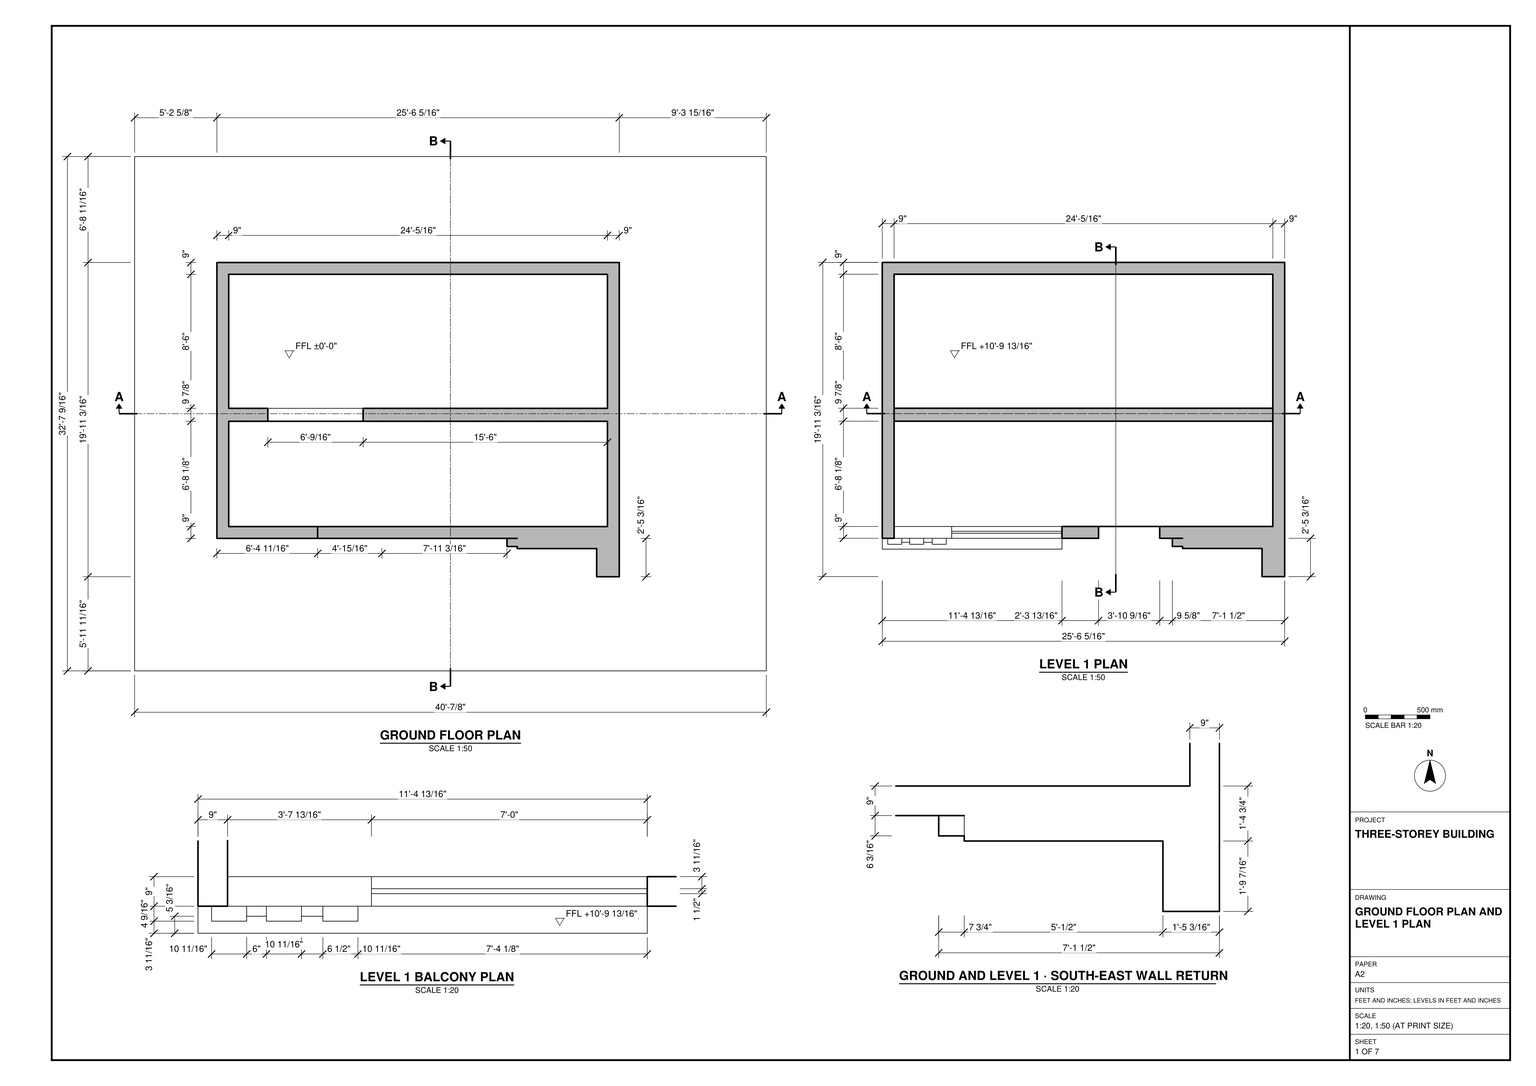
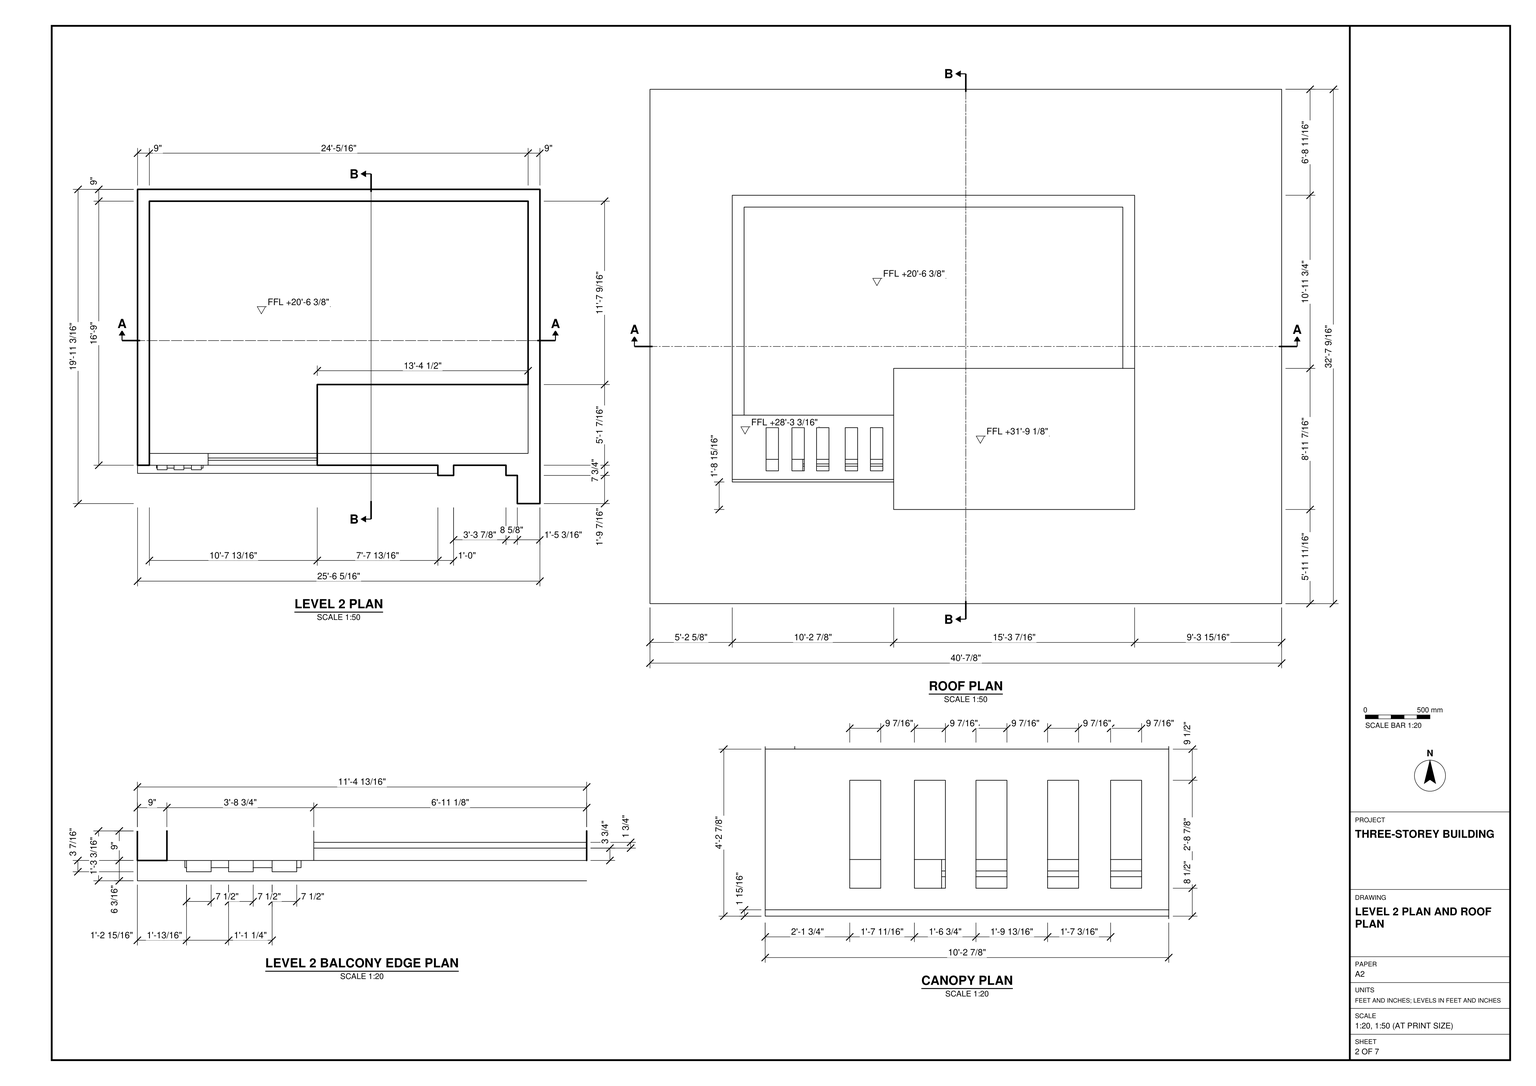
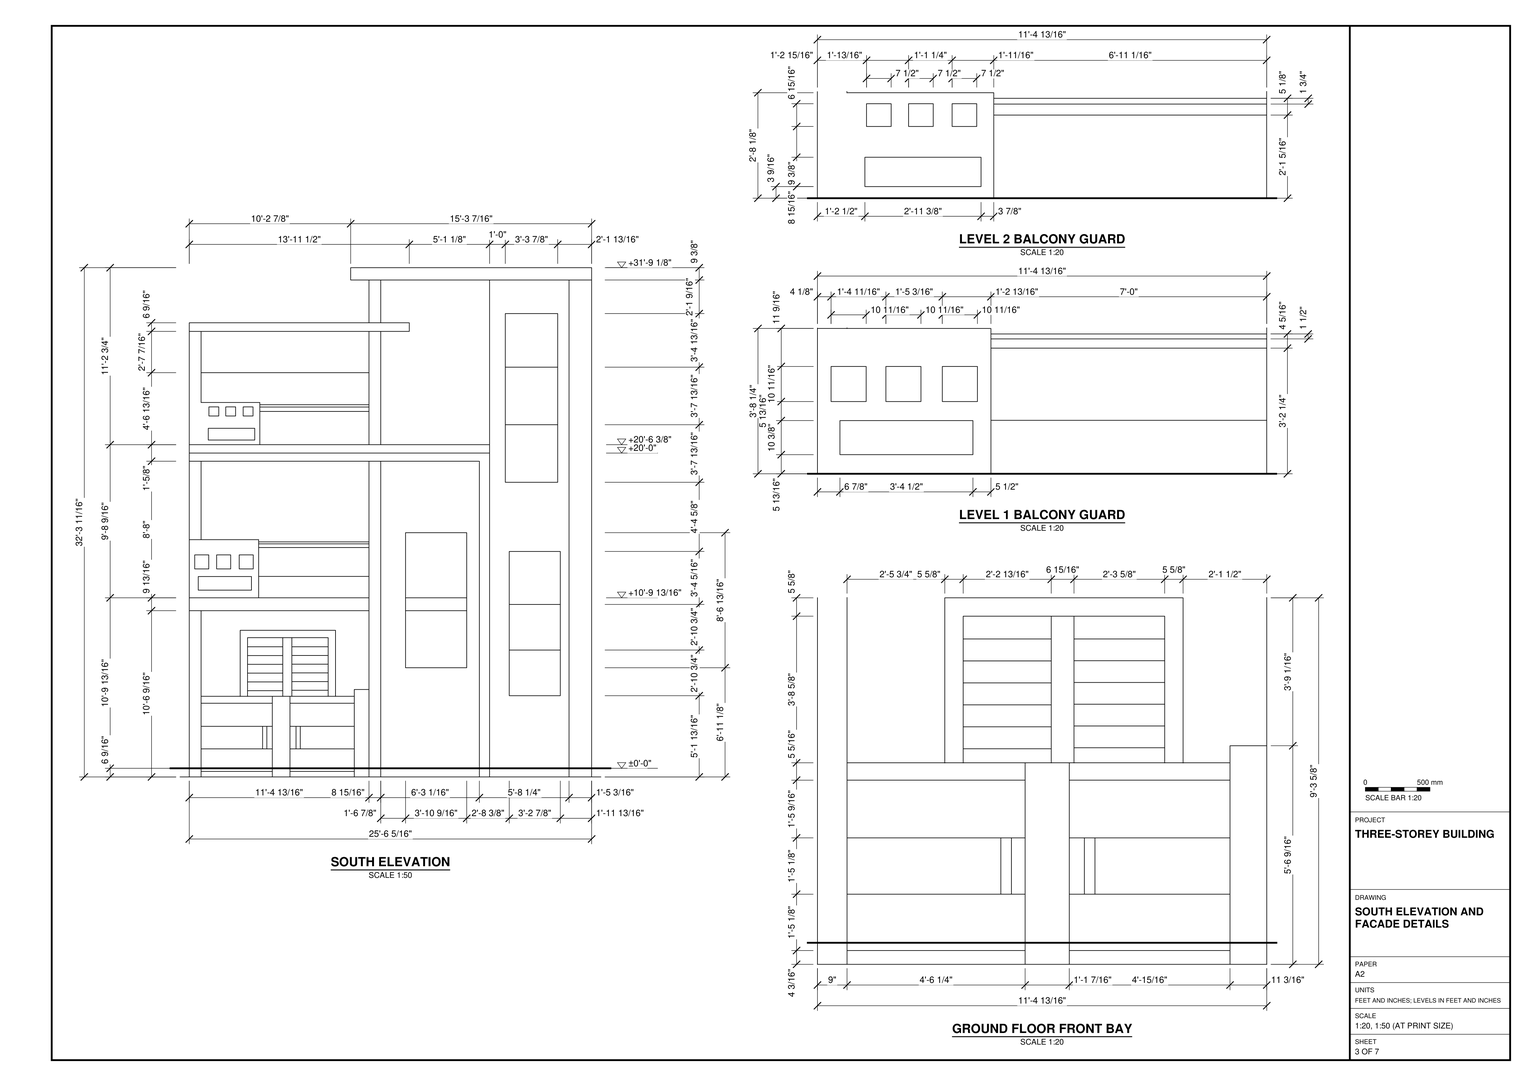
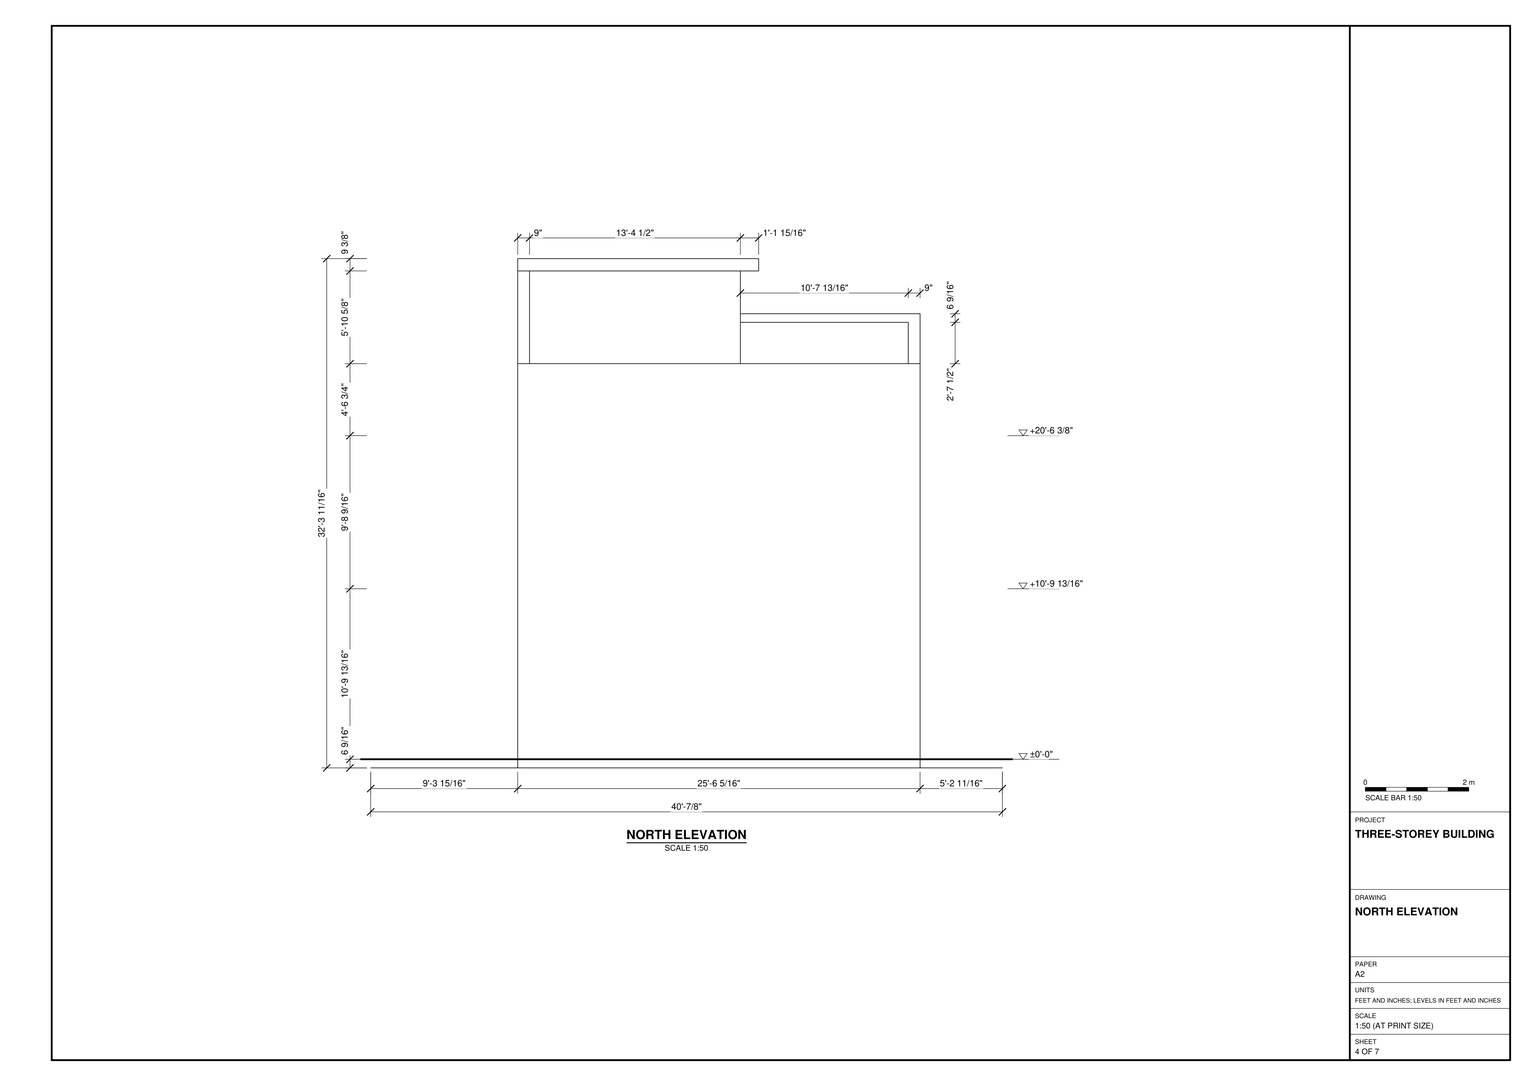
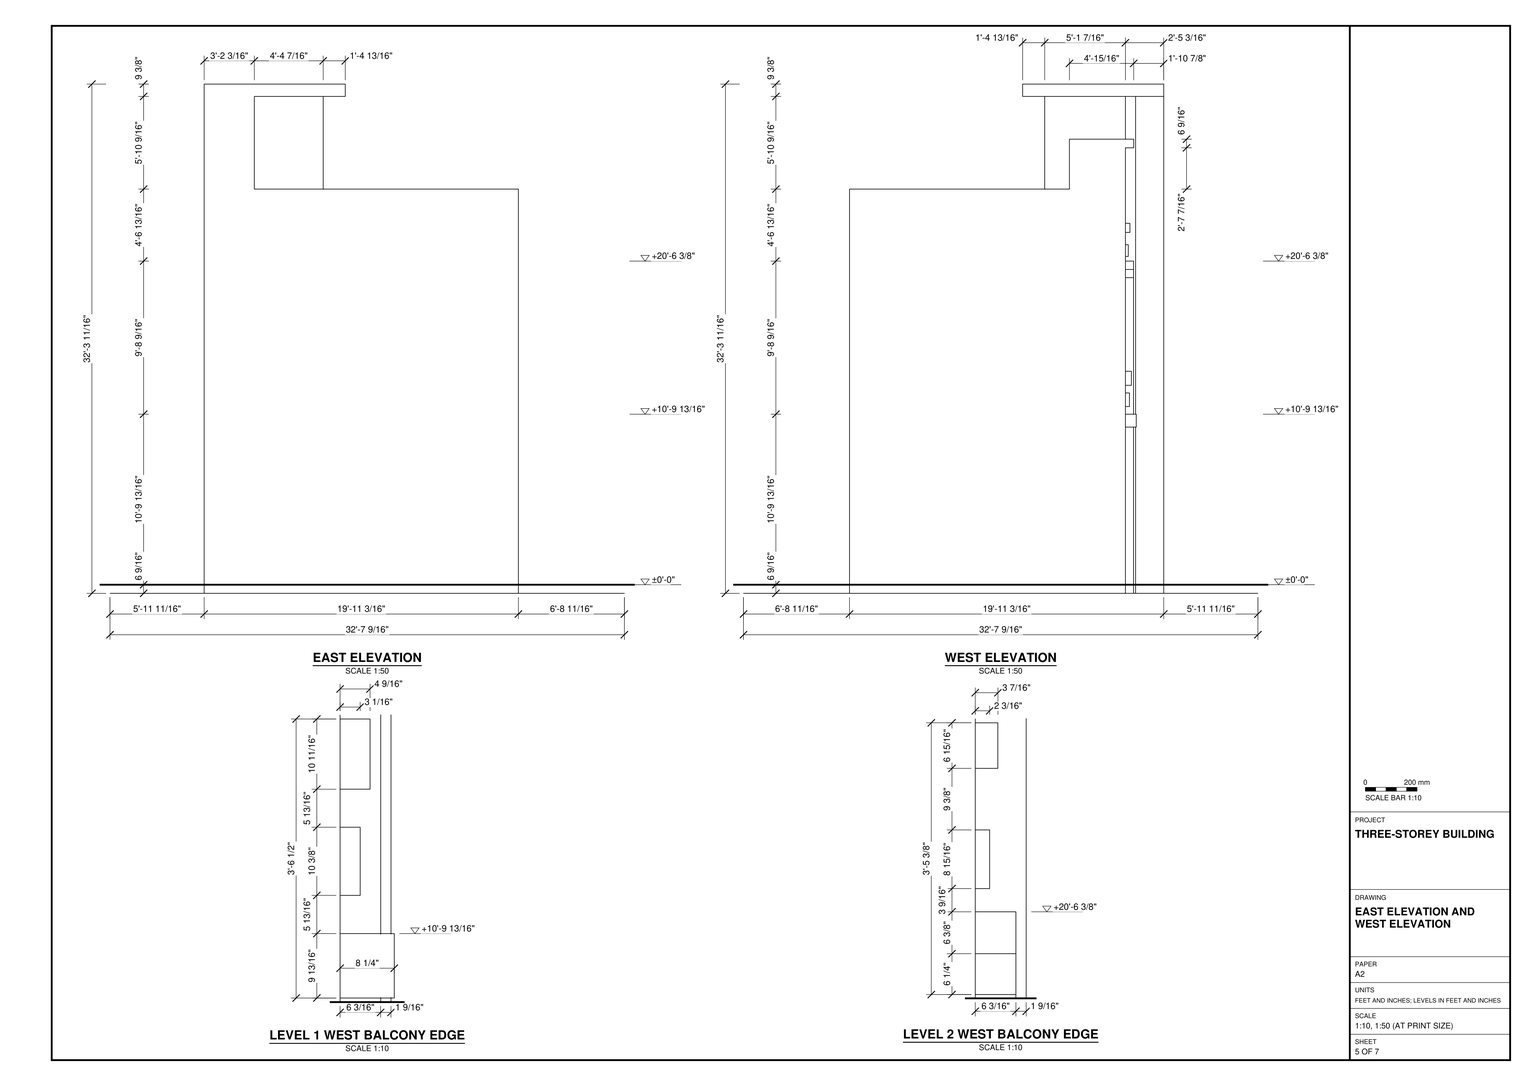
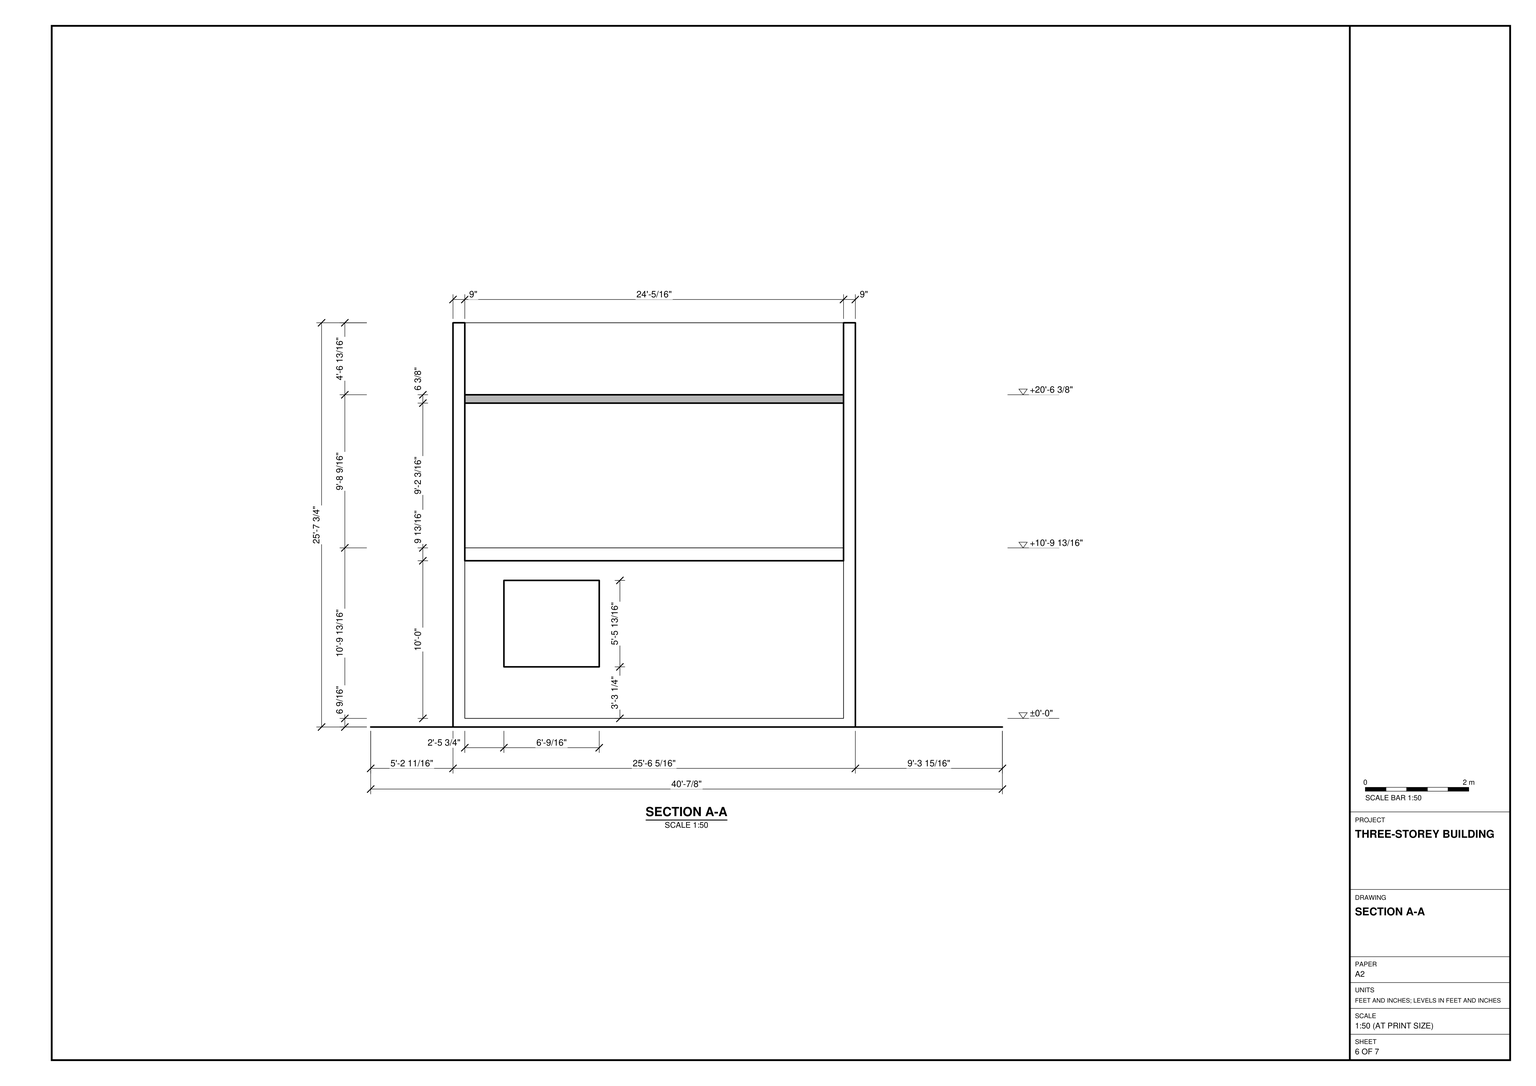
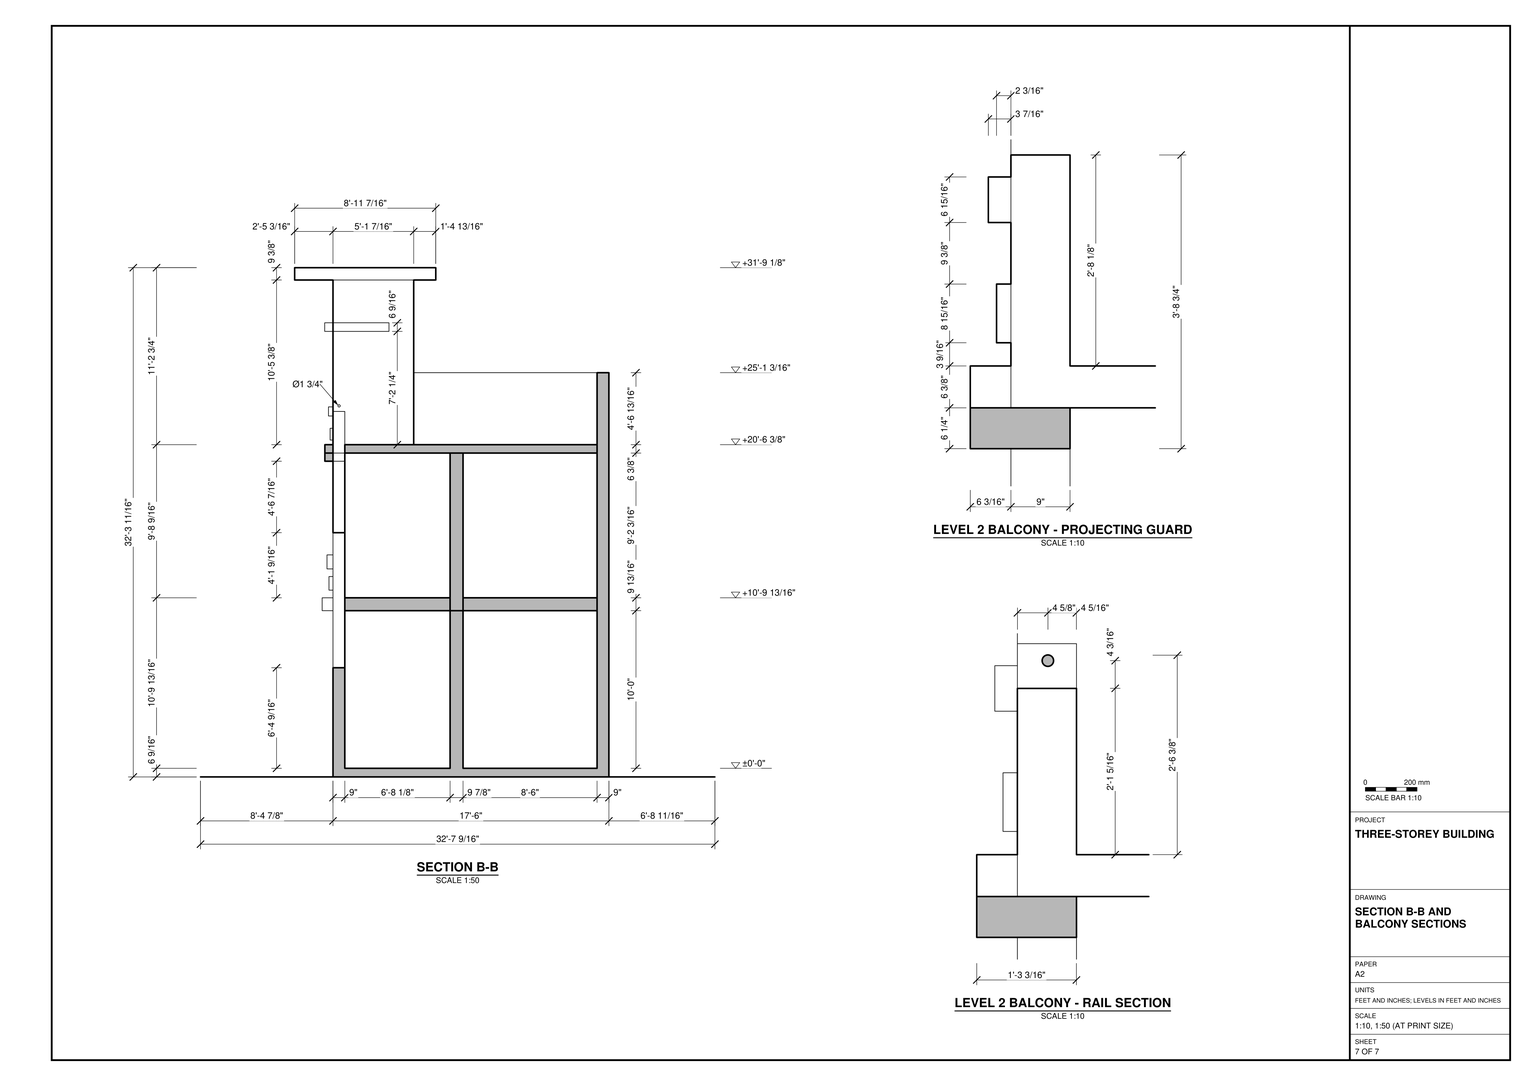
Build the three-storey building in SketchUp from task_files/diagram_01.pdf. Work in feet and inches. The overall model, including the rectangular base, measures 40'-7/8" along X, 32'-7 9/16" along Y and 32'-3 11/16" in height. Set the finished floor levels at ±0'-0", +10'-9 13/16" and +20'-6 3/8".

Position the smaller building footprint on the base using the setbacks on the ground floor plan. Model the floor slabs, perimeter walls and transverse walls at their drawn thicknesses. Keep the passage through the ground floor transverse wall and follow the stepped outline of the south-east wall return. Use the plans and elevations together to locate the openings and distinguish them from surface panels. Include stairs, built-in joinery and main furniture only where shown.

On the south face, align the stacked balconies above the ground floor front bay. Follow the separate guard details for each balcony rather than making the two guards identical. Model the lower slotted canopy and the higher flat roof over the south-east portion, leaving the top floor open where indicated in the roof plan.

Keep walls, slabs and roof elements in separate groups or components, and do the same for each furniture or joinery piece. Use components for repeated parts. Decor and loose items may be any suitable library components. Save one SketchUp model as output_files/three_storey_building_with_balconies_and_slotted_canopy.skp.

# SketchUp Ruby script. Lengths in inches.
U = 1.inch
M = Sketchup.active_model
def pt(a) = Geom::Point3d.new(a.map { |v| v * U })
def face(e, loops, mat)
  f = e.add_face(loops[0].map { |a| pt(a) })
  loops[1..].each { |l| e.add_face(l.map { |a| pt(a) }).erase! }
  f.material = f.back_material = mat if mat
  f
end
# faces: each face lists its corners as indices into pts; further lists are holes
def faces(e, pts, list, mat = nil) = list.each { |f| face(e, (f[0].is_a?(Array) ? f : [f]).map { |l| l.map { |i| pts[i] } }, mat) }
# xy, xz, yz: faces in a plane at the given z, y or x. An outline is a flat list of corners, or four numbers for a rectangle; further outlines are holes
def ring(l) = l.size == 4 ? [[l[0], l[1]], [l[2], l[1]], [l[2], l[3]], [l[0], l[3]]] : l.each_slice(2).to_a
def flat(e, list, mat, &to3) = list.each { |f| face(e, (f[0].is_a?(Array) ? f : [f]).map { |l| ring(l).map { |u, v| to3.(u, v) } }, mat) }
def xy(e, z, list, mat = nil) = flat(e, list, mat) { |x, y| [x, y, z] }
def xz(e, y, list, mat = nil) = flat(e, list, mat) { |x, z| [x, y, z] }
def yz(e, x, list, mat = nil) = flat(e, list, mat) { |y, z| [x, y, z] }
def lines(e, pts, list) = list.each { |a, b| e.add_line(pt(pts[a]), pt(pts[b])) }
# prism: a flat outline (further loops are holes) pulled along v
def prism(e, loops, v, mat = nil)
  f = face(e, loops, mat); d = Geom::Vector3d.new(v.map { |x| x * U })
  f.pushpull(f.normal.samedirection?(d) ? d.length : -d.length)
end
def box(e, o, s, mat = nil) = prism(e, [[o, [o[0] + s[0], o[1], o[2]], [o[0] + s[0], o[1] + s[1], o[2]], [o[0], o[1] + s[1], o[2]]]], [0, 0, s[2]], mat)
def at(x, y, z, deg = 0) = Geom::Transformation.translation(pt([x, y, z])) * Geom::Transformation.rotation(ORIGIN, Z_AXIS, deg.degrees)
def axes(o, x, y, z) = Geom::Transformation.new([*x, 0, *y, 0, *z, 0, *pt(o).to_a, 1])
def part(name) = M.definitions.add(name)
# library, detail: a bought-in or finely detailed component or shape, given as its bounding box
def library(name, o, s) = part(name).tap { |d| box(d.entities, o, s) }
def detail(e, o, s) = box(e.add_group.entities, o, s)
def put(e, d, t, mat = nil) = e.add_instance(d, t).tap { |i| i.material = mat if mat }
def group(e, t, mat = nil) = e.add_group.tap { |g| g.transformation = t; g.material = mat if mat }.entities
root = M.entities
M.materials.add("[Blinds Wood Light]").color = [155, 100, 14]
M.materials.add("[Carpet Diamond Olive]").color = [87, 77, 61]
M.materials.add("[Carpet Plush Charcoal]").color = [87, 87, 87]
M.materials.add("[Color M01]").color = [226, 226, 226]
M.materials.add("[Formica Beige]").color = [132, 117, 93]
M.materials.add("[Formica Beige]1").color = [255, 225, 180]
M.materials.add("[Formica Beige]2").color = [239, 212, 169]
M.materials.add("[Formica Beige]3").color = [211, 187, 149]
M.materials.add("[Formica Graystone]").color = [149, 146, 135]
M.materials.add("[Formica Laminate Dark]").color = [50, 53, 60]
M.materials.add("[Formica Speckled Grey]").color = [94, 105, 111]
M.materials.add("[Stone Masonry Multi]").color = [182, 175, 164]
M.materials.add("[Terrazzo Light Blue]").color = [196, 214, 227]
M.materials.add("[Translucent Glass Blue]").color = [100, 149, 237]
M.materials["[Translucent Glass Blue]"].alpha = 0.5
M.materials.add("[Translucent Glass Safety]").color = [204, 235, 244]
M.materials["[Translucent Glass Safety]"].alpha = 0.5
M.materials.add("[Translucent Glass Sky Reflection]").color = [126, 138, 183]
M.materials["[Translucent Glass Sky Reflection]"].alpha = 0.52
M.materials.add("[Wood Floor Light]").color = [204, 176, 127]
M.materials.add("[Wood Floor Parquet]").color = [145, 89, 39]
M.materials.add("[Wood Veneer 01]").color = [120, 70, 37]
xy(root,0,[[[0,0,480.875,391.5625],[351.76,71.67,368.96,71.67,368.96,310.89,62.65,310.89,62.65,100.86,283.48,100.86,283.48,94.67,291.26,94.67,291.26,93.11,351.76,93.11]],[351.76,71.67,351.76,93.11,291.26,93.11,291.26,100.86,62.65,100.86,62.65,310.89,368.96,310.89,368.96,71.67],[283.48,94.67,291.26,100.86]])
xy(root,6.5625,[[71.65,199.86,359.96,301.89]])
xy(root,6.5625,[[71.65,109.86,359.96,190]],"[Carpet Plush Charcoal]")
xy(root,45.8,[[101.42,190,173.98,199.86]])
xy(root,61.375,[[71.65,100.86,125.88,109.86],[125.88,100.86,139.33,109.86],[139.33,100.86,188.27,109.86]],"[Formica Laminate Dark]")
xy(root,61.83,[[306.24,93.11,345.12,100.86]],"[Formica Speckled Grey]")
xy(root,66.5625,[[188.27,100.86,199.46,109.86]],"[Formica Beige]1")
xy(root,83.12,[[227.29,100.86,273.85,109.86]],"[Formica Beige]")
xy(root,111.62,[[101.42,190,173.98,199.86]])
xy(root,126.5625,[[62.65,92.61,62.65,100.86,71.65,100.86,71.65,109.86,199.46,109.86,199.46,92.61],[71.65,109.86,359.96,190],[71.65,190,359.96,199.86],[71.65,199.86,359.96,301.89]])
xy(root,136.375,[[71.65,199.86,359.96,301.89]])
xy(root,136.375,[[71.65,109.86,359.96,190]],"[Carpet Diamond Olive]")
xy(root,136.375,[[62.65,92.61,199.46,100.86]],"[Formica Beige]1")
xy(root,142.19,[[69.5,97.79,110,100.86]])
xy(root,152.57,[[69.5,97.79,110,100.86]],"[Color M01]")
xy(root,158.36,[[66.8,96.29,77.49,100.86],[83.49,96.29,94.17,100.86],[100.67,96.29,111.36,100.86]])
xy(root,169.05,[[66.8,96.29,77.49,100.86],[83.49,96.29,94.17,100.86],[100.67,96.29,111.36,100.86]],"[Color M01]")
xy(root,171.65,[[306.24,93.11,345.12,100.86]],"[Formica Speckled Grey]")
xy(root,174.625,[[115.47,100.86,199.46,109.86]],"[Translucent Glass Safety]")
xy(root,180.625,[[71.65,100.86,115.47,109.86]],"[Formica Laminate Dark]")
xy(root,185.94,[[227.29,100.86,273.85,109.86]],"[Formica Beige]")
xy(root,224.3,[[303.25,93.11,343.12,100.86]],"[Formica Speckled Grey]")
xy(root,240.34,[[62.65,94.67,62.65,100.86,71.65,100.86,71.65,109.86,199.46,109.86,199.46,100.86,283.48,100.86,283.48,94.67]],"[Formica Beige]1")
xy(root,246.5625,[[62.65,94.67,291.26,94.67,291.26,100.86,199.46,100.86,199.46,109.86,71.65,109.86,71.65,100.86,62.65,100.86],[71.65,109.86,359.96,190],[71.65,190,359.96,199.86],[71.65,199.86,359.96,301.89]])
xy(root,252.9375,[[71.65,109.86,199.46,109.86,199.46,162.29,359.96,162.29,359.96,301.89,71.65,301.89],[199.46,109.86,359.96,162.29]])
xy(root,252.9375,[[62.65,94.67,291.26,100.86]],"[Formica Laminate Dark]")
xy(root,256.47,[[77.12,98.67,112.49,100.86]])
xy(root,265.41,[[77.12,98.67,112.49,100.86]],"[Color M01]")
xy(root,274.78,[[77.62,97.42,85.12,100.86],[90.43,97.42,97.93,100.86],[103.68,97.42,111.18,100.86]])
xy(root,278.25,[[116.37,100.86,199.46,109.86]],"[Translucent Glass Safety]")
xy(root,281.72,[[77.62,97.42,85.12,100.86],[90.43,97.42,97.93,100.86],[103.68,97.42,111.18,100.86]],"[Color M01]")
xy(root,285.0625,[[71.65,100.86,116.37,109.86]],"[Formica Laminate Dark]")
xy(root,307.75,[[359.96,109.86,368.96,109.86,368.96,310.89,62.65,310.89,62.65,143.48,71.65,143.48,71.65,301.89,359.96,301.89]],"[Formica Beige]3")
xy(root,339.18,[[[62.65,94.54,62.65,100.86,71.65,100.86,71.65,143.48,199.46,143.48,199.46,100.86,230.15,100.86,230.15,94.54],[88.39,101.1,97.83,133.98],[148.64,101.1,158.08,133.98],[126.83,101.1,136.27,133.98],[108.08,101.1,117.52,133.98],[167.83,101.1,177.27,133.98]]],"[Formica Laminate Dark]")
xy(root,345.75,[[[62.65,94.54,230.15,94.54,230.15,100.86,199.46,100.86,199.46,143.48,62.65,143.48],[88.39,101.1,97.83,133.98],[126.83,101.1,136.27,133.98],[148.64,101.1,158.08,133.98],[108.08,101.1,117.52,133.98],[167.83,101.1,177.27,133.98]]],"[Formica Laminate Dark]")
xy(root,352.74,[[303.25,93.11,343.12,100.86]])
xy(root,378.3,[[185.52,71.67,185.52,179.11,368.96,179.11,368.96,162.29,199.46,162.29,199.46,100.86,291.26,100.86,291.26,93.11,351.76,93.11,351.76,71.67],[359.96,109.86,368.96,162.29]],"[Formica Beige]3")
xy(root,387.6875,[[185.52,71.67,368.96,179.11]],"[Formica Beige]1")
xz(root,71.67,[[351.76,0,368.96,378.3],[185.52,378.3,368.96,387.6875]],"[Formica Beige]1")
xz(root,92.61,[[62.65,126.5625,199.46,136.375]],"[Formica Beige]1")
xz(root,93.11,[[[291.26,0,351.76,378.3],[303.25,224.3,343.12,352.74],[306.24,61.83,345.12,171.65]]],"[Formica Speckled Grey]")
xz(root,94.54,[[62.65,339.18,230.15,345.75]],"[Formica Laminate Dark]")
xz(root,94.67,[[283.48,0,291.26,0,291.26,246.5625,62.65,246.5625,62.65,240.34,283.48,240.34]],"[Formica Beige]1")
xz(root,94.67,[[62.65,246.5625,291.26,252.9375]],"[Formica Laminate Dark]")
xz(root,96.29,[[66.8,158.36,77.49,169.05],[83.49,158.36,94.17,169.05],[100.67,158.36,111.36,169.05]],"[Color M01]")
xz(root,97.42,[[77.62,274.78,85.12,281.72],[90.43,274.78,97.93,281.72],[103.68,274.78,111.18,281.72]],"[Color M01]")
xz(root,97.79,[[69.5,142.19,110,152.57]],"[Color M01]")
xz(root,98.67,[[77.12,256.47,112.49,265.41]],"[Color M01]")
xz(root,100.86,[[283.48,0,291.26,0,291.26,246.5625,208.43,246.5625,208.43,240.34,283.48,240.34],[62.65,240.34,71.65,246.5625],[199.46,240.34,208.43,246.5625],[199.46,246.5625,208.43,252.9375],[208.43,246.5625,291.26,252.9375],
  [199.46,339.18,208.43,345.75],[208.43,339.18,230.15,345.75]])
xz(root,100.86,[[[208.43,0,283.48,240.34],[227.29,83.12,273.85,185.94]],[208.43,252.9375,291.26,252.9375,291.26,378.3,208.43,378.3,208.43,345.75,230.15,345.75,230.15,339.18,208.43,339.18]],"[Blinds Wood Light]")
xz(root,100.86,[[62.65,0,71.65,126.5625],[188.27,0,199.46,66.5625],[115.47,136.375,199.46,152.65],[62.65,180.625,71.65,240.34]],"[Formica Beige]1")
xz(root,100.86,[[71.65,0,125.88,4.2],[125.88,0,139.33,61.375],[139.33,0,188.27,4.2],[118.48,21.36,121.71,38.51],[143.92,21.36,147.15,38.51],
  [71.65,56.09,125.88,61.375],[139.33,56.09,188.27,61.375],[[62.65,136.375,115.47,180.625],[69.5,142.19,110,152.57],[66.8,158.36,77.49,169.05],[100.67,158.36,111.36,169.05],[83.49,158.36,94.17,169.05]],[[62.65,252.9375,116.37,252.9375,116.37,285.0625,71.65,285.0625,71.65,339.18,62.65,339.18],[77.12,256.47,112.49,265.41],[90.43,274.78,97.93,281.72],[103.68,274.78,111.18,281.72],[77.62,274.78,85.12,281.72]]],"[Formica Laminate Dark]")
xz(root,100.86,[[115.47,152.65,199.46,174.625],[116.37,252.9375,199.46,278.25]],"[Translucent Glass Safety]")
xz(root,100.86,[[306.24,61.83,345.12,96.57],[306.24,96.57,345.12,131.31],[306.24,131.31,345.12,171.65],[303.25,224.3,343.12,268.12],[303.25,268.12,343.12,311.94],
  [303.25,311.94,343.12,352.74]],"[Translucent Glass Sky Reflection]")
xz(root,100.86,[[71.65,21.36,118.48,38.51],[121.71,21.36,125.88,38.51],[139.33,21.36,143.92,38.51],[147.15,21.36,188.27,38.51]],"[Wood Floor Light]")
xz(root,100.86,[[71.65,4.2,125.88,21.36],[139.33,4.2,188.27,21.36],[71.65,38.51,125.88,56.09],[139.33,38.51,188.27,56.09]],"[Wood Floor Parquet]")
xz(root,100.86,[[199.46,0,208.43,240.34],[199.46,252.9375,208.43,339.18],[199.46,345.75,208.43,378.3]],"[Wood Veneer 01]")
xz(root,101.1,[[88.39,339.18,97.83,345.75],[108.08,339.18,117.52,345.75],[126.83,339.18,136.27,345.75],[148.64,339.18,158.08,345.75],[167.83,339.18,177.27,345.75]])
xz(root,109.86,[[125.88,6.5625,139.33,61.375],[71.65,126.5625,199.46,136.375],[199.46,126.5625,227.29,136.375],[273.85,126.5625,359.96,136.375],[71.65,240.34,199.46,246.5625],
  [199.46,246.5625,359.96,252.9375]])
xz(root,109.86,[[227.29,83.12,273.85,126.5625],[227.29,126.5625,273.85,136.375],[227.29,136.375,273.85,185.94]],"[Formica Beige]")
xz(root,109.86,[[71.65,6.5625,125.88,61.375],[139.33,6.5625,188.27,61.375]],"[Formica Beige]1")
xz(root,109.86,[[188.27,6.5625,199.46,66.5625]],"[Formica Beige]2")
xz(root,109.86,[[359.96,307.75,368.96,378.3]],"[Formica Beige]3")
xz(root,109.86,[[71.65,252.9375,116.37,285.0625]],"[Formica Laminate Dark]")
xz(root,109.86,[[199.46,6.5625,199.46,126.5625,227.29,126.5625,227.29,83.12,273.85,83.12,273.85,126.5625,359.96,126.5625,359.96,6.5625],[199.46,136.375,199.46,246.5625,359.96,246.5625,359.96,136.375,273.85,136.375,273.85,185.94,227.29,185.94,227.29,136.375]],"[Stone Masonry Multi]")
xz(root,109.86,[[71.65,136.375,71.65,180.625,115.47,180.625,115.47,174.625,199.46,174.625,199.46,136.375],[116.37,252.9375,199.46,278.25]],"[Translucent Glass Safety]")
xz(root,133.98,[[88.39,339.18,97.83,345.75],[108.08,339.18,117.52,345.75],[126.83,339.18,136.27,345.75],[148.64,339.18,158.08,345.75],[167.83,339.18,177.27,345.75]])
xz(root,143.48,[[62.65,307.75,62.65,345.75,199.46,345.75,199.46,339.18,71.65,339.18,71.65,307.75]],"[Formica Beige]3")
xz(root,162.29,[[199.46,252.9375,359.96,378.3]],"[Formica Graystone]")
xz(root,179.11,[[185.52,378.3,368.96,387.6875]],"[Formica Beige]3")
xz(root,190,[[71.65,126.5625,359.96,136.375]])
xz(root,190,[[[101.42,45.8,173.98,111.62],[107.02,51.4,168.38,106.02]],[133.84,51.4,140.76,106.02]],"[Formica Laminate Dark]")
xz(root,190,[[[71.65,6.5625,359.96,126.5625],[101.42,45.8,173.98,111.62]],[71.65,136.375,359.96,246.5625]],"[Stone Masonry Multi]")
xz(root,190,[[107.02,51.4,133.84,58.52],[140.76,51.4,168.38,59.33],[107.02,58.52,133.84,65.65],[140.76,59.33,168.38,65.96],[107.02,65.65,133.84,72.33],
  [140.76,65.96,168.38,72.58],[107.02,72.33,133.84,79.02],[140.76,72.58,168.38,79.21],[107.02,79.02,133.84,85.71],[140.76,79.21,168.38,85.83],
  [107.02,85.71,133.84,92.4],[140.76,85.83,168.38,92.46],[107.02,92.4,133.84,99.08],[140.76,92.46,168.38,99.08],[107.02,99.08,133.84,106.02],
  [140.76,99.08,168.38,106.02]],"[Translucent Glass Blue]")
xz(root,199.86,[[[71.65,6.5625,359.96,126.5625],[101.42,45.8,173.98,111.62]],[71.65,126.5625,359.96,136.375],[71.65,136.375,359.96,246.5625]])
xz(root,301.89,[[71.65,6.5625,359.96,126.5625],[71.65,126.5625,359.96,136.375],[71.65,136.375,359.96,246.5625],[71.65,246.5625,359.96,252.9375]])
xz(root,301.89,[[71.65,252.9375,359.96,307.75]],"[Formica Graystone]")
xz(root,310.89,[[62.65,0,368.96,307.75]],"[Terrazzo Light Blue]")
yz(root,62.65,[[92.61,126.5625,100.86,136.375]],"[Formica Beige]1")
yz(root,62.65,[[94.67,240.34,100.86,246.5625]],"[Formica Beige]2")
yz(root,62.65,[[94.67,246.5625,100.86,252.9375]],"[Formica Laminate Dark]")
yz(root,62.65,[[100.86,0,100.86,339.18,94.54,339.18,94.54,345.75,143.48,345.75,143.48,307.75,310.89,307.75,310.89,0]],"[Terrazzo Light Blue]")
yz(root,66.8,[[96.29,158.36,100.86,169.05]])
yz(root,69.5,[[97.79,142.19,100.86,152.57]],"[Color M01]")
yz(root,71.65,[[199.86,6.5625,301.89,126.5625],[109.86,126.5625,190,136.375],[190,126.5625,199.86,246.5625],[199.86,126.5625,301.89,136.375],[199.86,136.375,301.89,246.5625],
  [100.86,240.34,109.86,246.5625],[190,246.5625,199.86,252.9375],[199.86,246.5625,301.89,252.9375]])
yz(root,71.65,[[100.86,180.625,109.86,240.34]],"[Formica Beige]1")
yz(root,71.65,[[100.86,61.375,109.86,126.5625]],"[Formica Beige]2")
yz(root,71.65,[[143.48,252.9375,301.89,307.75]],"[Formica Graystone]")
yz(root,71.65,[[109.86,252.9375,143.48,252.9375,143.48,339.18,100.86,339.18,100.86,285.0625,109.86,285.0625]],"[Formica Laminate Dark]")
yz(root,71.65,[[109.86,6.5625,190,126.5625],[109.86,136.375,190,246.5625]],"[Stone Masonry Multi]")
yz(root,77.12,[[98.67,256.47,100.86,265.41]],"[Color M01]")
yz(root,77.49,[[96.29,158.36,100.86,169.05]])
yz(root,77.62,[[97.42,274.78,100.86,281.72]],"[Color M01]")
yz(root,83.49,[[96.29,158.36,100.86,169.05]])
yz(root,85.12,[[97.42,274.78,100.86,281.72]],"[Color M01]")
yz(root,88.39,[[101.1,339.18,133.98,345.75]])
yz(root,90.43,[[97.42,274.78,100.86,281.72]],"[Color M01]")
yz(root,94.17,[[96.29,158.36,100.86,169.05]])
yz(root,97.83,[[101.1,339.18,133.98,345.75]])
yz(root,97.93,[[97.42,274.78,100.86,281.72]],"[Color M01]")
yz(root,100.67,[[96.29,158.36,100.86,169.05]])
yz(root,101.42,[[190,45.8,199.86,111.62]])
yz(root,103.68,[[97.42,274.78,100.86,281.72]],"[Color M01]")
yz(root,108.08,[[101.1,339.18,133.98,345.75]])
yz(root,110,[[97.79,142.19,100.86,152.57]],"[Color M01]")
yz(root,111.18,[[97.42,274.78,100.86,281.72]],"[Color M01]")
yz(root,111.36,[[96.29,158.36,100.86,169.05]])
yz(root,112.49,[[98.67,256.47,100.86,265.41]])
yz(root,115.47,[[[100.86,174.625,109.86,180.625],[105.43,177.44,105.24,177.47,105.06,177.55,104.9,177.66,104.78,177.82,104.71,178,104.68,178.19,104.71,178.39,104.78,178.57,104.9,178.73,105.06,178.84,105.24,178.92,105.43,178.94,105.625,178.92,105.81,178.84,105.96,178.73,106.08,178.57,106.16,178.39,106.18,178.19,106.16,178,106.08,177.82,105.96,177.66,105.81,177.55,105.625,177.47]]],"[Formica Laminate Dark]")
yz(root,116.37,[[[100.86,278.25,109.86,285.0625],[105.49,281.61,105.27,281.64,105.06,281.72,104.875,281.86,104.74,282.04,104.65,282.25,104.62,282.48,104.65,282.71,104.74,282.92,104.875,283.1,105.06,283.24,105.27,283.33,105.49,283.36,105.72,283.33,105.93,283.24,106.11,283.1,106.25,282.92,106.34,282.71,106.37,282.48,106.34,282.25,106.25,282.04,106.11,281.86,105.93,281.72,105.72,281.64]]],"[Formica Laminate Dark]")
yz(root,117.52,[[101.1,339.18,133.98,345.75]])
yz(root,126.83,[[101.1,339.18,133.98,345.75]])
yz(root,136.27,[[101.1,339.18,133.98,345.75]])
yz(root,139.33,[[100.86,6.5625,109.86,61.375]])
yz(root,148.64,[[101.1,339.18,133.98,345.75]])
yz(root,158.08,[[101.1,339.18,133.98,345.75]])
yz(root,167.83,[[101.1,339.18,133.98,345.75]])
yz(root,173.98,[[190,45.8,199.86,111.62]])
yz(root,177.27,[[101.1,339.18,133.98,345.75]])
yz(root,185.52,[[71.67,378.3,179.11,387.6875]],"[Formica Beige]1")
yz(root,188.27,[[100.86,61.375,109.86,66.5625]],"[Formica Beige]1")
yz(root,199.46,[[100.86,126.5625,109.86,174.625],[100.86,240.34,109.86,246.5625],[100.86,246.5625,109.86,278.25],[100.86,339.18,143.48,345.75]])
yz(root,199.46,[[92.61,126.5625,100.86,136.375],[[100.86,174.625,109.86,240.34],[105.43,177.44,105.625,177.47,105.81,177.55,105.96,177.66,106.08,177.82,106.16,178,106.18,178.19,106.16,178.39,106.08,178.57,105.96,178.73,105.81,178.84,105.625,178.92,105.43,178.94,105.24,178.92,105.06,178.84,104.9,178.73,104.78,178.57,104.71,178.39,104.68,178.19,104.71,178,104.78,177.82,104.9,177.66,105.06,177.55,105.24,177.47]],[[109.86,252.9375,109.86,278.25,100.86,278.25,100.86,339.18,143.48,339.18,143.48,345.75,100.86,345.75,100.86,378.3,162.29,378.3,162.29,252.9375],[105.49,281.61,105.72,281.64,105.93,281.72,106.11,281.86,106.25,282.04,106.34,282.25,106.37,282.48,106.34,282.71,106.25,282.92,106.11,283.1,105.93,283.24,105.72,283.33,105.49,283.36,105.27,283.33,105.06,283.24,104.875,283.1,104.74,282.92,104.65,282.71,104.62,282.48,104.65,282.25,104.74,282.04,104.875,281.86,105.06,281.72,105.27,281.64]]],"[Formica Beige]1")
yz(root,199.46,[[100.86,66.5625,109.86,126.5625]],"[Formica Beige]2")
yz(root,227.29,[[100.86,83.12,109.86,185.94]],"[Formica Beige]")
yz(root,230.15,[[94.54,339.18,100.86,345.75]],"[Formica Laminate Dark]")
yz(root,273.85,[[100.86,83.12,109.86,185.94]],"[Formica Beige]")
yz(root,283.48,[[94.67,0,100.86,240.34]],"[Formica Beige]1")
yz(root,291.26,[[93.11,0,93.11,378.3,100.86,378.3,100.86,252.9375,94.67,252.9375,94.67,0]],"[Formica Speckled Grey]")
yz(root,303.25,[[93.11,224.3,100.86,268.12],[93.11,268.12,100.86,311.94],[93.11,311.94,100.86,352.74]],"[Formica Speckled Grey]")
yz(root,306.24,[[93.11,61.83,100.86,96.57],[93.11,96.57,100.86,131.31],[93.11,131.31,100.86,171.65]],"[Formica Speckled Grey]")
yz(root,343.12,[[93.11,224.3,100.86,268.12],[93.11,268.12,100.86,311.94],[93.11,311.94,100.86,352.74]],"[Formica Speckled Grey]")
yz(root,345.12,[[93.11,61.83,100.86,96.57],[93.11,96.57,100.86,131.31],[93.11,131.31,100.86,171.65]],"[Formica Speckled Grey]")
yz(root,351.76,[[71.67,0,93.11,378.3]],"[Formica Beige]1")
yz(root,359.96,[[199.86,6.5625,301.89,126.5625],[190,126.5625,199.86,246.5625],[199.86,126.5625,301.89,136.375],[199.86,136.375,301.89,246.5625],[109.86,246.5625,190,252.9375],
  [190,246.5625,199.86,252.9375],[199.86,246.5625,301.89,252.9375]])
yz(root,359.96,[[162.29,252.9375,301.89,307.75],[109.86,307.75,162.29,378.3]],"[Formica Graystone]")
yz(root,359.96,[[109.86,6.5625,190,126.5625],[109.86,136.375,190,246.5625]],"[Stone Masonry Multi]")
yz(root,368.96,[[71.67,0,310.89,0,310.89,307.75,109.86,307.75,109.86,378.3,179.11,378.3,179.11,387.6875,71.67,387.6875]],"[Terrazzo Light Blue]")
p = [[115.47,105.24,177.47],[115.47,105.43,177.44],[199.46,105.43,177.44],[199.46,105.24,177.47],[115.47,105.625,177.47],[199.46,105.625,177.47],
  [115.47,104.9,177.66],[115.47,105.06,177.55],[199.46,105.06,177.55],[199.46,104.9,177.66],[115.47,105.81,177.55],[199.46,105.81,177.55],
  [115.47,105.96,177.66],[199.46,105.96,177.66],[115.47,104.78,177.82],[199.46,104.78,177.82],[115.47,106.08,177.82],[199.46,106.08,177.82],
  [115.47,104.71,178],[199.46,104.71,178],[115.47,106.16,178],[199.46,106.16,178],[115.47,104.68,178.19],[199.46,104.68,178.19],
  [115.47,106.18,178.19],[199.46,106.18,178.19],[115.47,104.71,178.39],[199.46,104.71,178.39],[115.47,106.16,178.39],[199.46,106.16,178.39],
  [115.47,104.78,178.57],[199.46,104.78,178.57],[115.47,106.08,178.57],[199.46,106.08,178.57],[115.47,104.9,178.73],[199.46,104.9,178.73],
  [115.47,105.96,178.73],[199.46,105.96,178.73],[115.47,105.06,178.84],[199.46,105.06,178.84],[115.47,105.81,178.84],[199.46,105.81,178.84],
  [115.47,105.24,178.92],[199.46,105.24,178.92],[115.47,105.625,178.92],[199.46,105.625,178.92],[115.47,105.43,178.94],[199.46,105.43,178.94],
  [116.37,105.06,281.72],[116.37,105.27,281.64],[199.46,105.27,281.64],[199.46,105.06,281.72],[116.37,105.49,281.61],[199.46,105.49,281.61],
  [116.37,105.72,281.64],[199.46,105.72,281.64],[116.37,105.93,281.72],[199.46,105.93,281.72],[116.37,104.875,281.86],[199.46,104.875,281.86],
  [116.37,106.11,281.86],[199.46,106.11,281.86],[116.37,104.74,282.04],[199.46,104.74,282.04],[116.37,106.25,282.04],[199.46,106.25,282.04],
  [116.37,104.65,282.25],[199.46,104.65,282.25],[116.37,106.34,282.25],[199.46,106.34,282.25],[116.37,104.62,282.48],[199.46,104.62,282.48],
  [116.37,106.37,282.48],[199.46,106.37,282.48],[116.37,104.65,282.71],[199.46,104.65,282.71],[116.37,106.34,282.71],[199.46,106.34,282.71],
  [116.37,104.74,282.92],[199.46,104.74,282.92],[116.37,106.25,282.92],[199.46,106.25,282.92],[116.37,104.875,283.1],[199.46,104.875,283.1],
  [116.37,106.11,283.1],[199.46,106.11,283.1],[116.37,105.06,283.24],[199.46,105.06,283.24],[116.37,105.93,283.24],[199.46,105.93,283.24],
  [116.37,105.27,283.33],[199.46,105.27,283.33],[116.37,105.72,283.33],[199.46,105.72,283.33],[116.37,105.49,283.36],[199.46,105.49,283.36],
  [188.27,100.86,6.5625],[188.27,109.86,6.5625]]
faces(root,p,[[0,1,2,3],[1,4,5,2],[6,7,8,9],[7,0,3,8],[4,10,11,5],[10,12,13,11],[14,6,9,15],[12,16,17,13],
  [18,14,15,19],[16,20,21,17],[22,18,19,23],[20,24,25,21],[26,22,23,27],[24,28,29,25],[30,26,27,31],[28,32,33,29],
  [34,30,31,35],[32,36,37,33],[38,34,35,39],[36,40,41,37],[42,38,39,43],[40,44,45,41],[46,42,43,47],[44,46,47,45],
  [48,49,50,51],[49,52,53,50],[52,54,55,53],[54,56,57,55],[58,48,51,59],[56,60,61,57],[62,58,59,63],[60,64,65,61],
  [66,62,63,67],[64,68,69,65],[70,66,67,71],[68,72,73,69],[74,70,71,75],[72,76,77,73],[78,74,75,79],[76,80,81,77],
  [82,78,79,83],[80,84,85,81],[86,82,83,87],[84,88,89,85],[90,86,87,91],[88,92,93,89],[94,90,91,95],[92,94,95,93]],"[Formica Laminate Dark]")
lines(root,p,[[96,97]])
